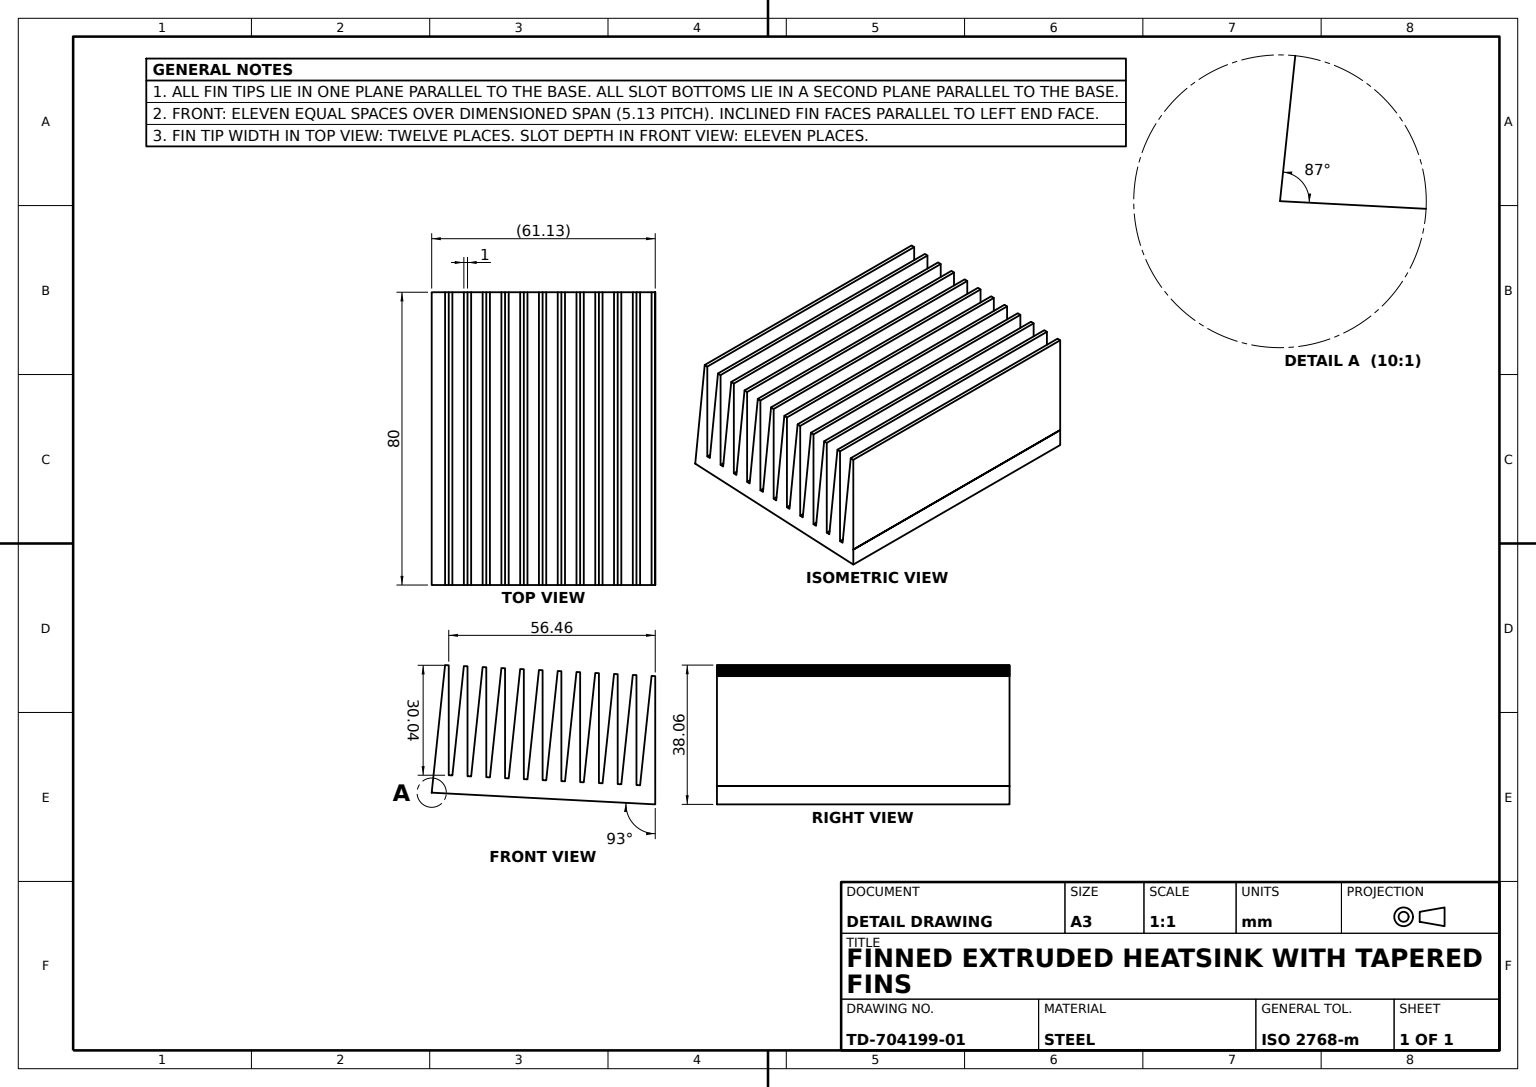
ISO-10303-21;
HEADER;
FILE_DESCRIPTION((''),'2;1');
FILE_NAME('','',(''),(''),'','','');
FILE_SCHEMA(('AUTOMOTIVE_DESIGN'));
ENDSEC;
DATA;
#1=APPLICATION_CONTEXT('');
#2=PRODUCT_CONTEXT('',#1,'mechanical');
#3=PRODUCT('','','',(#2));
#4=PRODUCT_DEFINITION_FORMATION('','',#3);
#5=PRODUCT_DEFINITION_CONTEXT('',#1,'design');
#6=PRODUCT_DEFINITION('','',#4,#5);
#7=PRODUCT_DEFINITION_SHAPE('','',#6);
#8=(LENGTH_UNIT()NAMED_UNIT(*)SI_UNIT(.MILLI.,.METRE.));
#9=(NAMED_UNIT(*)PLANE_ANGLE_UNIT()SI_UNIT($,.RADIAN.));
#10=(NAMED_UNIT(*)SI_UNIT($,.STERADIAN.)SOLID_ANGLE_UNIT());
#11=UNCERTAINTY_MEASURE_WITH_UNIT(LENGTH_MEASURE(1.E-05),#8,'distance_accuracy_value','');
#12=(GEOMETRIC_REPRESENTATION_CONTEXT(3)GLOBAL_UNCERTAINTY_ASSIGNED_CONTEXT((#11))GLOBAL_UNIT_ASSIGNED_CONTEXT((#8,#9,#10))REPRESENTATION_CONTEXT('',''));
#13=CARTESIAN_POINT('',(-19.094272,35.,40.));
#14=VERTEX_POINT('',#13);
#15=CARTESIAN_POINT('',(-19.094272,35.,-40.));
#16=VERTEX_POINT('',#15);
#17=CARTESIAN_POINT('',(-19.094272,35.,0.));
#18=DIRECTION('',(0.,0.,-1.));
#19=VECTOR('',#18,1000.);
#20=LINE('',#17,#19);
#21=EDGE_CURVE('',#14,#16,#20,.T.);
#22=ORIENTED_EDGE('',*,*,#21,.F.);
#23=CARTESIAN_POINT('',(-18.094272,35.,40.));
#24=VERTEX_POINT('',#23);
#25=CARTESIAN_POINT('',(-31.21,35.,40.));
#26=DIRECTION('',(1.,0.,0.));
#27=VECTOR('',#26,1000.);
#28=LINE('',#25,#27);
#29=EDGE_CURVE('',#14,#24,#28,.T.);
#30=ORIENTED_EDGE('',*,*,#29,.T.);
#31=CARTESIAN_POINT('',(-18.094272,35.,-40.));
#32=VERTEX_POINT('',#31);
#33=CARTESIAN_POINT('',(-18.094272,35.,0.));
#34=DIRECTION('',(0.,0.,1.));
#35=VECTOR('',#34,1000.);
#36=LINE('',#33,#35);
#37=EDGE_CURVE('',#32,#24,#36,.T.);
#38=ORIENTED_EDGE('',*,*,#37,.F.);
#39=CARTESIAN_POINT('',(-31.21,35.,-40.));
#40=DIRECTION('',(-1.,0.,0.));
#41=VECTOR('',#40,1000.);
#42=LINE('',#39,#41);
#43=EDGE_CURVE('',#32,#16,#42,.T.);
#44=ORIENTED_EDGE('',*,*,#43,.T.);
#45=EDGE_LOOP('',(#22,#30,#38,#44));
#46=FACE_OUTER_BOUND('',#45,.T.);
#47=CARTESIAN_POINT('',(0.,35.,0.));
#48=DIRECTION('',(0.,-1.,0.));
#49=AXIS2_PLACEMENT_3D('',#47,#48,#18);
#50=PLANE('',#49);
#51=ADVANCED_FACE('',(#46),#50,.F.);
#52=CARTESIAN_POINT('',(27.165728,35.,40.));
#53=VERTEX_POINT('',#52);
#54=CARTESIAN_POINT('',(25.593494,5.,40.));
#55=VERTEX_POINT('',#54);
#56=CARTESIAN_POINT('',(25.262071,-1.323929,40.));
#57=DIRECTION('',(-0.052335956,-0.998629535,0.));
#58=VECTOR('',#57,1000.);
#59=LINE('',#56,#58);
#60=EDGE_CURVE('',#53,#55,#59,.T.);
#61=ORIENTED_EDGE('',*,*,#60,.F.);
#62=CARTESIAN_POINT('',(27.165728,35.,-40.));
#63=VERTEX_POINT('',#62);
#64=CARTESIAN_POINT('',(27.165728,35.,0.));
#65=LINE('',#64,#19);
#66=EDGE_CURVE('',#53,#63,#65,.T.);
#67=ORIENTED_EDGE('',*,*,#66,.T.);
#68=CARTESIAN_POINT('',(25.593494,5.,-40.));
#69=VERTEX_POINT('',#68);
#70=CARTESIAN_POINT('',(27.005834,31.949037,-40.));
#71=LINE('',#70,#58);
#72=EDGE_CURVE('',#63,#69,#71,.T.);
#73=ORIENTED_EDGE('',*,*,#72,.T.);
#74=CARTESIAN_POINT('',(25.593494,5.,-65.));
#75=LINE('',#74,#35);
#76=EDGE_CURVE('',#69,#55,#75,.T.);
#77=ORIENTED_EDGE('',*,*,#76,.T.);
#78=EDGE_LOOP('',(#61,#67,#73,#77));
#79=FACE_OUTER_BOUND('',#78,.T.);
#80=CARTESIAN_POINT('',(25.262071,-1.323929,-65.));
#81=DIRECTION('',(-0.998629535,0.052335956,0.));
#82=AXIS2_PLACEMENT_3D('',#80,#81,#57);
#83=PLANE('',#82);
#84=ADVANCED_FACE('',(#79),#83,.T.);
#85=CARTESIAN_POINT('',(7.605728,35.,-40.));
#86=VERTEX_POINT('',#85);
#87=CARTESIAN_POINT('',(7.605728,35.,40.));
#88=VERTEX_POINT('',#87);
#89=CARTESIAN_POINT('',(7.605728,35.,0.));
#90=LINE('',#89,#35);
#91=EDGE_CURVE('',#86,#88,#90,.T.);
#92=ORIENTED_EDGE('',*,*,#91,.T.);
#93=CARTESIAN_POINT('',(9.177961,5.,40.));
#94=VERTEX_POINT('',#93);
#95=DIRECTION('',(-0.052335956,0.998629535,0.));
#96=VECTOR('',#95,1000.);
#97=LINE('',#93,#96);
#98=EDGE_CURVE('',#94,#88,#97,.T.);
#99=ORIENTED_EDGE('',*,*,#98,.F.);
#100=CARTESIAN_POINT('',(9.177961,5.,-40.));
#101=VERTEX_POINT('',#100);
#102=CARTESIAN_POINT('',(9.177961,5.,-65.));
#103=LINE('',#102,#35);
#104=EDGE_CURVE('',#101,#94,#103,.T.);
#105=ORIENTED_EDGE('',*,*,#104,.F.);
#106=CARTESIAN_POINT('',(7.499409,37.028674,-40.));
#107=LINE('',#106,#96);
#108=EDGE_CURVE('',#101,#86,#107,.T.);
#109=ORIENTED_EDGE('',*,*,#108,.T.);
#110=EDGE_LOOP('',(#92,#99,#105,#109));
#111=FACE_OUTER_BOUND('',#110,.T.);
#112=DIRECTION('',(0.998629535,0.052335956,0.));
#113=AXIS2_PLACEMENT_3D('',#102,#112,#95);
#114=PLANE('',#113);
#115=ADVANCED_FACE('',(#111),#114,.T.);
#116=CARTESIAN_POINT('',(1.465728,35.,-40.));
#117=VERTEX_POINT('',#116);
#118=CARTESIAN_POINT('',(-0.106506,5.,-40.));
#119=VERTEX_POINT('',#118);
#120=CARTESIAN_POINT('',(1.376227,33.292228,-40.));
#121=LINE('',#120,#58);
#122=EDGE_CURVE('',#117,#119,#121,.T.);
#123=ORIENTED_EDGE('',*,*,#122,.T.);
#124=CARTESIAN_POINT('',(-0.106506,5.,40.));
#125=VERTEX_POINT('',#124);
#126=CARTESIAN_POINT('',(-0.106506,5.,-65.));
#127=LINE('',#126,#35);
#128=EDGE_CURVE('',#119,#125,#127,.T.);
#129=ORIENTED_EDGE('',*,*,#128,.T.);
#130=CARTESIAN_POINT('',(1.465728,35.,40.));
#131=VERTEX_POINT('',#130);
#132=CARTESIAN_POINT('',(-0.367535,0.019262,40.));
#133=LINE('',#132,#58);
#134=EDGE_CURVE('',#131,#125,#133,.T.);
#135=ORIENTED_EDGE('',*,*,#134,.F.);
#136=CARTESIAN_POINT('',(1.465728,35.,0.));
#137=LINE('',#136,#19);
#138=EDGE_CURVE('',#131,#117,#137,.T.);
#139=ORIENTED_EDGE('',*,*,#138,.T.);
#140=EDGE_LOOP('',(#123,#129,#135,#139));
#141=FACE_OUTER_BOUND('',#140,.T.);
#142=CARTESIAN_POINT('',(-0.367535,0.019262,-65.));
#143=AXIS2_PLACEMENT_3D('',#142,#81,#57);
#144=PLANE('',#143);
#145=ADVANCED_FACE('',(#141),#144,.T.);
#146=CARTESIAN_POINT('',(24.597961,5.,-40.));
#147=VERTEX_POINT('',#146);
#148=CARTESIAN_POINT('',(-31.21,5.,-40.));
#149=LINE('',#148,#27);
#150=EDGE_CURVE('',#147,#69,#149,.T.);
#151=ORIENTED_EDGE('',*,*,#150,.F.);
#152=CARTESIAN_POINT('',(24.597961,5.,40.));
#153=VERTEX_POINT('',#152);
#154=CARTESIAN_POINT('',(24.597961,5.,-65.));
#155=LINE('',#154,#35);
#156=EDGE_CURVE('',#147,#153,#155,.T.);
#157=ORIENTED_EDGE('',*,*,#156,.T.);
#158=CARTESIAN_POINT('',(0.,5.,40.));
#159=LINE('',#158,#27);
#160=EDGE_CURVE('',#153,#55,#159,.T.);
#161=ORIENTED_EDGE('',*,*,#160,.T.);
#162=ORIENTED_EDGE('',*,*,#76,.F.);
#163=EDGE_LOOP('',(#151,#157,#161,#162));
#164=FACE_OUTER_BOUND('',#163,.T.);
#165=CARTESIAN_POINT('',(0.,5.,-65.));
#166=AXIS2_PLACEMENT_3D('',#165,#48,#18);
#167=PLANE('',#166);
#168=ADVANCED_FACE('',(#164),#167,.F.);
#169=CARTESIAN_POINT('',(-21.662039,5.,40.));
#170=VERTEX_POINT('',#169);
#171=CARTESIAN_POINT('',(-23.234272,35.,40.));
#172=VERTEX_POINT('',#171);
#173=CARTESIAN_POINT('',(-21.341384,-1.118455,40.));
#174=LINE('',#173,#96);
#175=EDGE_CURVE('',#170,#172,#174,.T.);
#176=ORIENTED_EDGE('',*,*,#175,.F.);
#177=CARTESIAN_POINT('',(-21.662039,5.,-40.));
#178=VERTEX_POINT('',#177);
#179=CARTESIAN_POINT('',(-21.662039,5.,-65.));
#180=LINE('',#179,#35);
#181=EDGE_CURVE('',#178,#170,#180,.T.);
#182=ORIENTED_EDGE('',*,*,#181,.F.);
#183=CARTESIAN_POINT('',(-23.234272,35.,-40.));
#184=VERTEX_POINT('',#183);
#185=CARTESIAN_POINT('',(-23.256118,35.416845,-40.));
#186=LINE('',#185,#96);
#187=EDGE_CURVE('',#178,#184,#186,.T.);
#188=ORIENTED_EDGE('',*,*,#187,.T.);
#189=CARTESIAN_POINT('',(-23.234272,35.,0.));
#190=LINE('',#189,#35);
#191=EDGE_CURVE('',#184,#172,#190,.T.);
#192=ORIENTED_EDGE('',*,*,#191,.T.);
#193=EDGE_LOOP('',(#176,#182,#188,#192));
#194=FACE_OUTER_BOUND('',#193,.T.);
#195=CARTESIAN_POINT('',(-21.341384,-1.118455,-65.));
#196=AXIS2_PLACEMENT_3D('',#195,#112,#95);
#197=PLANE('',#196);
#198=ADVANCED_FACE('',(#194),#197,.T.);
#199=ORIENTED_EDGE('',*,*,#128,.F.);
#200=CARTESIAN_POINT('',(-1.102039,5.,-40.));
#201=VERTEX_POINT('',#200);
#202=LINE('',#148,#41);
#203=EDGE_CURVE('',#119,#201,#202,.T.);
#204=ORIENTED_EDGE('',*,*,#203,.T.);
#205=CARTESIAN_POINT('',(-1.102039,5.,40.));
#206=VERTEX_POINT('',#205);
#207=CARTESIAN_POINT('',(-1.102039,5.,-65.));
#208=LINE('',#207,#35);
#209=EDGE_CURVE('',#201,#206,#208,.T.);
#210=ORIENTED_EDGE('',*,*,#209,.T.);
#211=LINE('',#158,#41);
#212=EDGE_CURVE('',#125,#206,#211,.T.);
#213=ORIENTED_EDGE('',*,*,#212,.F.);
#214=EDGE_LOOP('',(#199,#204,#210,#213));
#215=FACE_OUTER_BOUND('',#214,.T.);
#216=DIRECTION('',(0.,1.,0.));
#217=AXIS2_PLACEMENT_3D('',#165,#216,#40);
#218=PLANE('',#217);
#219=ADVANCED_FACE('',(#215),#218,.T.);
#220=CARTESIAN_POINT('',(4.037961,5.,-40.));
#221=VERTEX_POINT('',#220);
#222=CARTESIAN_POINT('',(4.037961,5.,40.));
#223=VERTEX_POINT('',#222);
#224=CARTESIAN_POINT('',(4.037961,5.,-65.));
#225=LINE('',#224,#35);
#226=EDGE_CURVE('',#221,#223,#225,.T.);
#227=ORIENTED_EDGE('',*,*,#226,.F.);
#228=CARTESIAN_POINT('',(2.465728,35.,-40.));
#229=VERTEX_POINT('',#228);
#230=CARTESIAN_POINT('',(2.373488,36.760036,-40.));
#231=LINE('',#230,#96);
#232=EDGE_CURVE('',#221,#229,#231,.T.);
#233=ORIENTED_EDGE('',*,*,#232,.T.);
#234=CARTESIAN_POINT('',(2.465728,35.,40.));
#235=VERTEX_POINT('',#234);
#236=CARTESIAN_POINT('',(2.465728,35.,0.));
#237=LINE('',#236,#35);
#238=EDGE_CURVE('',#229,#235,#237,.T.);
#239=ORIENTED_EDGE('',*,*,#238,.T.);
#240=CARTESIAN_POINT('',(4.288222,0.224736,40.));
#241=LINE('',#240,#96);
#242=EDGE_CURVE('',#223,#235,#241,.T.);
#243=ORIENTED_EDGE('',*,*,#242,.F.);
#244=EDGE_LOOP('',(#227,#233,#239,#243));
#245=FACE_OUTER_BOUND('',#244,.T.);
#246=CARTESIAN_POINT('',(4.288222,0.224736,-65.));
#247=AXIS2_PLACEMENT_3D('',#246,#112,#95);
#248=PLANE('',#247);
#249=ADVANCED_FACE('',(#245),#248,.T.);
#250=CARTESIAN_POINT('',(-11.382039,5.,-40.));
#251=VERTEX_POINT('',#250);
#252=CARTESIAN_POINT('',(-11.382039,5.,40.));
#253=VERTEX_POINT('',#252);
#254=CARTESIAN_POINT('',(-11.382039,5.,-65.));
#255=LINE('',#254,#35);
#256=EDGE_CURVE('',#251,#253,#255,.T.);
#257=ORIENTED_EDGE('',*,*,#256,.F.);
#258=CARTESIAN_POINT('',(-12.954272,35.,-40.));
#259=VERTEX_POINT('',#258);
#260=CARTESIAN_POINT('',(-13.004276,35.954122,-40.));
#261=LINE('',#260,#96);
#262=EDGE_CURVE('',#251,#259,#261,.T.);
#263=ORIENTED_EDGE('',*,*,#262,.T.);
#264=CARTESIAN_POINT('',(-12.954272,35.,40.));
#265=VERTEX_POINT('',#264);
#266=CARTESIAN_POINT('',(-12.954272,35.,0.));
#267=LINE('',#266,#35);
#268=EDGE_CURVE('',#259,#265,#267,.T.);
#269=ORIENTED_EDGE('',*,*,#268,.T.);
#270=CARTESIAN_POINT('',(-11.089542,-0.581178,40.));
#271=LINE('',#270,#96);
#272=EDGE_CURVE('',#253,#265,#271,.T.);
#273=ORIENTED_EDGE('',*,*,#272,.F.);
#274=EDGE_LOOP('',(#257,#263,#269,#273));
#275=FACE_OUTER_BOUND('',#274,.T.);
#276=CARTESIAN_POINT('',(-11.089542,-0.581178,-65.));
#277=AXIS2_PLACEMENT_3D('',#276,#112,#95);
#278=PLANE('',#277);
#279=ADVANCED_FACE('',(#275),#278,.T.);
#280=CARTESIAN_POINT('',(-10.386506,5.,40.));
#281=VERTEX_POINT('',#280);
#282=EDGE_CURVE('',#281,#253,#211,.T.);
#283=ORIENTED_EDGE('',*,*,#282,.F.);
#284=CARTESIAN_POINT('',(-10.386506,5.,-40.));
#285=VERTEX_POINT('',#284);
#286=CARTESIAN_POINT('',(-10.386506,5.,-65.));
#287=LINE('',#286,#35);
#288=EDGE_CURVE('',#285,#281,#287,.T.);
#289=ORIENTED_EDGE('',*,*,#288,.F.);
#290=EDGE_CURVE('',#285,#251,#202,.T.);
#291=ORIENTED_EDGE('',*,*,#290,.T.);
#292=ORIENTED_EDGE('',*,*,#256,.T.);
#293=EDGE_LOOP('',(#283,#289,#291,#292));
#294=FACE_OUTER_BOUND('',#293,.T.);
#295=ADVANCED_FACE('',(#294),#218,.T.);
#296=CARTESIAN_POINT('',(-25.806506,5.,-40.));
#297=VERTEX_POINT('',#296);
#298=CARTESIAN_POINT('',(-26.802039,5.,-40.));
#299=VERTEX_POINT('',#298);
#300=EDGE_CURVE('',#297,#299,#202,.T.);
#301=ORIENTED_EDGE('',*,*,#300,.T.);
#302=CARTESIAN_POINT('',(-26.802039,5.,40.));
#303=VERTEX_POINT('',#302);
#304=CARTESIAN_POINT('',(-26.802039,5.,-65.));
#305=LINE('',#304,#35);
#306=EDGE_CURVE('',#299,#303,#305,.T.);
#307=ORIENTED_EDGE('',*,*,#306,.T.);
#308=CARTESIAN_POINT('',(-25.806506,5.,40.));
#309=VERTEX_POINT('',#308);
#310=LINE('',#308,#41);
#311=EDGE_CURVE('',#309,#303,#310,.T.);
#312=ORIENTED_EDGE('',*,*,#311,.F.);
#313=CARTESIAN_POINT('',(-25.806506,5.,-65.));
#314=LINE('',#313,#35);
#315=EDGE_CURVE('',#297,#309,#314,.T.);
#316=ORIENTED_EDGE('',*,*,#315,.F.);
#317=EDGE_LOOP('',(#301,#307,#312,#316));
#318=FACE_OUTER_BOUND('',#317,.T.);
#319=AXIS2_PLACEMENT_3D('',#313,#216,#40);
#320=PLANE('',#319);
#321=ADVANCED_FACE('',(#318),#320,.T.);
#322=CARTESIAN_POINT('',(5.033494,5.,-40.));
#323=VERTEX_POINT('',#322);
#324=CARTESIAN_POINT('',(5.033494,5.,40.));
#325=VERTEX_POINT('',#324);
#326=CARTESIAN_POINT('',(5.033494,5.,-65.));
#327=LINE('',#326,#35);
#328=EDGE_CURVE('',#323,#325,#327,.T.);
#329=ORIENTED_EDGE('',*,*,#328,.F.);
#330=EDGE_CURVE('',#323,#221,#202,.T.);
#331=ORIENTED_EDGE('',*,*,#330,.T.);
#332=ORIENTED_EDGE('',*,*,#226,.T.);
#333=EDGE_CURVE('',#325,#223,#211,.T.);
#334=ORIENTED_EDGE('',*,*,#333,.F.);
#335=EDGE_LOOP('',(#329,#331,#332,#334));
#336=FACE_OUTER_BOUND('',#335,.T.);
#337=ADVANCED_FACE('',(#336),#218,.T.);
#338=CARTESIAN_POINT('',(-24.234272,35.,-40.));
#339=VERTEX_POINT('',#338);
#340=CARTESIAN_POINT('',(-24.253379,34.635419,-40.));
#341=LINE('',#340,#58);
#342=EDGE_CURVE('',#339,#297,#341,.T.);
#343=ORIENTED_EDGE('',*,*,#342,.T.);
#344=ORIENTED_EDGE('',*,*,#315,.T.);
#345=CARTESIAN_POINT('',(-24.234272,35.,40.));
#346=VERTEX_POINT('',#345);
#347=LINE('',#345,#58);
#348=EDGE_CURVE('',#346,#309,#347,.T.);
#349=ORIENTED_EDGE('',*,*,#348,.F.);
#350=CARTESIAN_POINT('',(-24.234272,35.,0.));
#351=LINE('',#350,#19);
#352=EDGE_CURVE('',#346,#339,#351,.T.);
#353=ORIENTED_EDGE('',*,*,#352,.T.);
#354=EDGE_LOOP('',(#343,#344,#349,#353));
#355=FACE_OUTER_BOUND('',#354,.T.);
#356=CARTESIAN_POINT('',(-24.234272,35.,-65.));
#357=AXIS2_PLACEMENT_3D('',#356,#81,#57);
#358=PLANE('',#357);
#359=ADVANCED_FACE('',(#355),#358,.T.);
#360=CARTESIAN_POINT('',(-28.374272,35.,-40.));
#361=VERTEX_POINT('',#360);
#362=CARTESIAN_POINT('',(-28.382039,35.148207,-40.));
#363=LINE('',#362,#96);
#364=EDGE_CURVE('',#299,#361,#363,.T.);
#365=ORIENTED_EDGE('',*,*,#364,.T.);
#366=CARTESIAN_POINT('',(-28.374272,35.,40.));
#367=VERTEX_POINT('',#366);
#368=CARTESIAN_POINT('',(-28.374272,35.,0.));
#369=LINE('',#368,#35);
#370=EDGE_CURVE('',#361,#367,#369,.T.);
#371=ORIENTED_EDGE('',*,*,#370,.T.);
#372=LINE('',#302,#96);
#373=EDGE_CURVE('',#303,#367,#372,.T.);
#374=ORIENTED_EDGE('',*,*,#373,.F.);
#375=ORIENTED_EDGE('',*,*,#306,.F.);
#376=EDGE_LOOP('',(#365,#371,#374,#375));
#377=FACE_OUTER_BOUND('',#376,.T.);
#378=AXIS2_PLACEMENT_3D('',#304,#112,#95);
#379=PLANE('',#378);
#380=ADVANCED_FACE('',(#377),#379,.T.);
#381=CARTESIAN_POINT('',(-2.674272,35.,-40.));
#382=VERTEX_POINT('',#381);
#383=CARTESIAN_POINT('',(-2.752433,36.491398,-40.));
#384=LINE('',#383,#96);
#385=EDGE_CURVE('',#201,#382,#384,.T.);
#386=ORIENTED_EDGE('',*,*,#385,.T.);
#387=CARTESIAN_POINT('',(-2.674272,35.,40.));
#388=VERTEX_POINT('',#387);
#389=CARTESIAN_POINT('',(-2.674272,35.,0.));
#390=LINE('',#389,#35);
#391=EDGE_CURVE('',#382,#388,#390,.T.);
#392=ORIENTED_EDGE('',*,*,#391,.T.);
#393=CARTESIAN_POINT('',(-0.837699,-0.043902,40.));
#394=LINE('',#393,#96);
#395=EDGE_CURVE('',#206,#388,#394,.T.);
#396=ORIENTED_EDGE('',*,*,#395,.F.);
#397=ORIENTED_EDGE('',*,*,#209,.F.);
#398=EDGE_LOOP('',(#386,#392,#396,#397));
#399=FACE_OUTER_BOUND('',#398,.T.);
#400=CARTESIAN_POINT('',(-0.837699,-0.043902,-65.));
#401=AXIS2_PLACEMENT_3D('',#400,#112,#95);
#402=PLANE('',#401);
#403=ADVANCED_FACE('',(#399),#402,.T.);
#404=CARTESIAN_POINT('',(-6.242039,5.,40.));
#405=VERTEX_POINT('',#404);
#406=CARTESIAN_POINT('',(-7.814272,35.,40.));
#407=VERTEX_POINT('',#406);
#408=CARTESIAN_POINT('',(-5.96362,-0.31254,40.));
#409=LINE('',#408,#96);
#410=EDGE_CURVE('',#405,#407,#409,.T.);
#411=ORIENTED_EDGE('',*,*,#410,.F.);
#412=CARTESIAN_POINT('',(-6.242039,5.,-40.));
#413=VERTEX_POINT('',#412);
#414=CARTESIAN_POINT('',(-6.242039,5.,-65.));
#415=LINE('',#414,#35);
#416=EDGE_CURVE('',#413,#405,#415,.T.);
#417=ORIENTED_EDGE('',*,*,#416,.F.);
#418=CARTESIAN_POINT('',(-7.814272,35.,-40.));
#419=VERTEX_POINT('',#418);
#420=CARTESIAN_POINT('',(-7.878354,36.22276,-40.));
#421=LINE('',#420,#96);
#422=EDGE_CURVE('',#413,#419,#421,.T.);
#423=ORIENTED_EDGE('',*,*,#422,.T.);
#424=CARTESIAN_POINT('',(-7.814272,35.,0.));
#425=LINE('',#424,#35);
#426=EDGE_CURVE('',#419,#407,#425,.T.);
#427=ORIENTED_EDGE('',*,*,#426,.T.);
#428=EDGE_LOOP('',(#411,#417,#423,#427));
#429=FACE_OUTER_BOUND('',#428,.T.);
#430=CARTESIAN_POINT('',(-5.96362,-0.31254,-65.));
#431=AXIS2_PLACEMENT_3D('',#430,#112,#95);
#432=PLANE('',#431);
#433=ADVANCED_FACE('',(#429),#432,.T.);
#434=CARTESIAN_POINT('',(-8.814272,35.,40.));
#435=VERTEX_POINT('',#434);
#436=EDGE_CURVE('',#435,#407,#28,.T.);
#437=ORIENTED_EDGE('',*,*,#436,.T.);
#438=ORIENTED_EDGE('',*,*,#426,.F.);
#439=CARTESIAN_POINT('',(-8.814272,35.,-40.));
#440=VERTEX_POINT('',#439);
#441=EDGE_CURVE('',#419,#440,#42,.T.);
#442=ORIENTED_EDGE('',*,*,#441,.T.);
#443=CARTESIAN_POINT('',(-8.814272,35.,0.));
#444=LINE('',#443,#19);
#445=EDGE_CURVE('',#435,#440,#444,.T.);
#446=ORIENTED_EDGE('',*,*,#445,.F.);
#447=EDGE_LOOP('',(#437,#438,#442,#446));
#448=FACE_OUTER_BOUND('',#447,.T.);
#449=ADVANCED_FACE('',(#448),#50,.F.);
#450=CARTESIAN_POINT('',(-10.619378,0.556538,40.));
#451=LINE('',#450,#58);
#452=EDGE_CURVE('',#435,#281,#451,.T.);
#453=ORIENTED_EDGE('',*,*,#452,.F.);
#454=ORIENTED_EDGE('',*,*,#445,.T.);
#455=CARTESIAN_POINT('',(-8.875615,33.829504,-40.));
#456=LINE('',#455,#58);
#457=EDGE_CURVE('',#440,#285,#456,.T.);
#458=ORIENTED_EDGE('',*,*,#457,.T.);
#459=ORIENTED_EDGE('',*,*,#288,.T.);
#460=EDGE_LOOP('',(#453,#454,#458,#459));
#461=FACE_OUTER_BOUND('',#460,.T.);
#462=CARTESIAN_POINT('',(-10.619378,0.556538,-65.));
#463=AXIS2_PLACEMENT_3D('',#462,#81,#57);
#464=PLANE('',#463);
#465=ADVANCED_FACE('',(#461),#464,.T.);
#466=CARTESIAN_POINT('',(6.605728,35.,40.));
#467=VERTEX_POINT('',#466);
#468=EDGE_CURVE('',#467,#88,#28,.T.);
#469=ORIENTED_EDGE('',*,*,#468,.T.);
#470=ORIENTED_EDGE('',*,*,#91,.F.);
#471=CARTESIAN_POINT('',(6.605728,35.,-40.));
#472=VERTEX_POINT('',#471);
#473=EDGE_CURVE('',#86,#472,#42,.T.);
#474=ORIENTED_EDGE('',*,*,#473,.T.);
#475=CARTESIAN_POINT('',(6.605728,35.,0.));
#476=LINE('',#475,#19);
#477=EDGE_CURVE('',#467,#472,#476,.T.);
#478=ORIENTED_EDGE('',*,*,#477,.F.);
#479=EDGE_LOOP('',(#469,#470,#474,#478));
#480=FACE_OUTER_BOUND('',#479,.T.);
#481=ADVANCED_FACE('',(#480),#50,.F.);
#482=CARTESIAN_POINT('',(4.758386,-0.249376,40.));
#483=LINE('',#482,#58);
#484=EDGE_CURVE('',#467,#325,#483,.T.);
#485=ORIENTED_EDGE('',*,*,#484,.F.);
#486=ORIENTED_EDGE('',*,*,#477,.T.);
#487=CARTESIAN_POINT('',(6.502148,33.02359,-40.));
#488=LINE('',#487,#58);
#489=EDGE_CURVE('',#472,#323,#488,.T.);
#490=ORIENTED_EDGE('',*,*,#489,.T.);
#491=ORIENTED_EDGE('',*,*,#328,.T.);
#492=EDGE_LOOP('',(#485,#486,#490,#491));
#493=FACE_OUTER_BOUND('',#492,.T.);
#494=CARTESIAN_POINT('',(4.758386,-0.249376,-65.));
#495=AXIS2_PLACEMENT_3D('',#494,#81,#57);
#496=PLANE('',#495);
#497=ADVANCED_FACE('',(#493),#496,.T.);
#498=CARTESIAN_POINT('',(19.457961,5.,-40.));
#499=VERTEX_POINT('',#498);
#500=CARTESIAN_POINT('',(19.457961,5.,40.));
#501=VERTEX_POINT('',#500);
#502=CARTESIAN_POINT('',(19.457961,5.,-65.));
#503=LINE('',#502,#35);
#504=EDGE_CURVE('',#499,#501,#503,.T.);
#505=ORIENTED_EDGE('',*,*,#504,.T.);
#506=CARTESIAN_POINT('',(20.453494,5.,40.));
#507=VERTEX_POINT('',#506);
#508=LINE('',#506,#41);
#509=EDGE_CURVE('',#507,#501,#508,.T.);
#510=ORIENTED_EDGE('',*,*,#509,.F.);
#511=CARTESIAN_POINT('',(20.453494,5.,-40.));
#512=VERTEX_POINT('',#511);
#513=CARTESIAN_POINT('',(20.453494,5.,-65.));
#514=LINE('',#513,#35);
#515=EDGE_CURVE('',#512,#507,#514,.T.);
#516=ORIENTED_EDGE('',*,*,#515,.F.);
#517=EDGE_CURVE('',#512,#499,#202,.T.);
#518=ORIENTED_EDGE('',*,*,#517,.T.);
#519=EDGE_LOOP('',(#505,#510,#516,#518));
#520=FACE_OUTER_BOUND('',#519,.T.);
#521=AXIS2_PLACEMENT_3D('',#513,#216,#40);
#522=PLANE('',#521);
#523=ADVANCED_FACE('',(#520),#522,.T.);
#524=CARTESIAN_POINT('',(16.885728,35.,-40.));
#525=VERTEX_POINT('',#524);
#526=CARTESIAN_POINT('',(15.313494,5.,-40.));
#527=VERTEX_POINT('',#526);
#528=CARTESIAN_POINT('',(16.753991,32.486314,-40.));
#529=LINE('',#528,#58);
#530=EDGE_CURVE('',#525,#527,#529,.T.);
#531=ORIENTED_EDGE('',*,*,#530,.T.);
#532=CARTESIAN_POINT('',(15.313494,5.,40.));
#533=VERTEX_POINT('',#532);
#534=CARTESIAN_POINT('',(15.313494,5.,-65.));
#535=LINE('',#534,#35);
#536=EDGE_CURVE('',#527,#533,#535,.T.);
#537=ORIENTED_EDGE('',*,*,#536,.T.);
#538=CARTESIAN_POINT('',(16.885728,35.,40.));
#539=VERTEX_POINT('',#538);
#540=LINE('',#538,#58);
#541=EDGE_CURVE('',#539,#533,#540,.T.);
#542=ORIENTED_EDGE('',*,*,#541,.F.);
#543=CARTESIAN_POINT('',(16.885728,35.,0.));
#544=LINE('',#543,#19);
#545=EDGE_CURVE('',#539,#525,#544,.T.);
#546=ORIENTED_EDGE('',*,*,#545,.T.);
#547=EDGE_LOOP('',(#531,#537,#542,#546));
#548=FACE_OUTER_BOUND('',#547,.T.);
#549=CARTESIAN_POINT('',(16.885728,35.,-65.));
#550=AXIS2_PLACEMENT_3D('',#549,#81,#57);
#551=PLANE('',#550);
#552=ADVANCED_FACE('',(#548),#551,.T.);
#553=CARTESIAN_POINT('',(17.885728,35.,-40.));
#554=VERTEX_POINT('',#553);
#555=CARTESIAN_POINT('',(17.885728,35.,40.));
#556=VERTEX_POINT('',#555);
#557=CARTESIAN_POINT('',(17.885728,35.,0.));
#558=LINE('',#557,#35);
#559=EDGE_CURVE('',#554,#556,#558,.T.);
#560=ORIENTED_EDGE('',*,*,#559,.T.);
#561=LINE('',#500,#96);
#562=EDGE_CURVE('',#501,#556,#561,.T.);
#563=ORIENTED_EDGE('',*,*,#562,.F.);
#564=ORIENTED_EDGE('',*,*,#504,.F.);
#565=CARTESIAN_POINT('',(17.751252,37.56595,-40.));
#566=LINE('',#565,#96);
#567=EDGE_CURVE('',#499,#554,#566,.T.);
#568=ORIENTED_EDGE('',*,*,#567,.T.);
#569=EDGE_LOOP('',(#560,#563,#564,#568));
#570=FACE_OUTER_BOUND('',#569,.T.);
#571=AXIS2_PLACEMENT_3D('',#502,#112,#95);
#572=PLANE('',#571);
#573=ADVANCED_FACE('',(#570),#572,.T.);
#574=CARTESIAN_POINT('',(-30.947753,5.,40.));
#575=VERTEX_POINT('',#574);
#576=CARTESIAN_POINT('',(-30.947753,5.,-40.));
#577=VERTEX_POINT('',#576);
#578=CARTESIAN_POINT('',(-30.947753,5.,-65.));
#579=LINE('',#578,#19);
#580=EDGE_CURVE('',#575,#577,#579,.T.);
#581=ORIENTED_EDGE('',*,*,#580,.T.);
#582=CARTESIAN_POINT('',(-31.21,0.,-40.));
#583=VERTEX_POINT('',#582);
#584=CARTESIAN_POINT('',(-29.379308,34.903981,-40.));
#585=DIRECTION('',(0.05237737,0.998627364,0.));
#586=VECTOR('',#585,1000.);
#587=LINE('',#584,#586);
#588=EDGE_CURVE('',#583,#577,#587,.T.);
#589=ORIENTED_EDGE('',*,*,#588,.F.);
#590=CARTESIAN_POINT('',(-31.21,0.,40.));
#591=VERTEX_POINT('',#590);
#592=LINE('',#590,#35);
#593=EDGE_CURVE('',#583,#591,#592,.T.);
#594=ORIENTED_EDGE('',*,*,#593,.T.);
#595=CARTESIAN_POINT('',(-29.374272,35.,40.));
#596=LINE('',#595,#586);
#597=EDGE_CURVE('',#591,#575,#596,.T.);
#598=ORIENTED_EDGE('',*,*,#597,.T.);
#599=EDGE_LOOP('',(#581,#589,#594,#598));
#600=FACE_OUTER_BOUND('',#599,.T.);
#601=CARTESIAN_POINT('',(-29.374272,35.,-140.145));
#602=DIRECTION('',(0.998627364,-0.05237737,0.));
#603=AXIS2_PLACEMENT_3D('',#601,#602,#585);
#604=PLANE('',#603);
#605=ADVANCED_FACE('',(#600),#604,.F.);
#606=CARTESIAN_POINT('',(-13.954272,35.,-40.));
#607=VERTEX_POINT('',#606);
#608=CARTESIAN_POINT('',(-15.526506,5.,-40.));
#609=VERTEX_POINT('',#608);
#610=CARTESIAN_POINT('',(-14.001537,34.098143,-40.));
#611=LINE('',#610,#58);
#612=EDGE_CURVE('',#607,#609,#611,.T.);
#613=ORIENTED_EDGE('',*,*,#612,.T.);
#614=CARTESIAN_POINT('',(-15.526506,5.,40.));
#615=VERTEX_POINT('',#614);
#616=CARTESIAN_POINT('',(-15.526506,5.,-65.));
#617=LINE('',#616,#35);
#618=EDGE_CURVE('',#609,#615,#617,.T.);
#619=ORIENTED_EDGE('',*,*,#618,.T.);
#620=CARTESIAN_POINT('',(-13.954272,35.,40.));
#621=VERTEX_POINT('',#620);
#622=LINE('',#620,#58);
#623=EDGE_CURVE('',#621,#615,#622,.T.);
#624=ORIENTED_EDGE('',*,*,#623,.F.);
#625=CARTESIAN_POINT('',(-13.954272,35.,0.));
#626=LINE('',#625,#19);
#627=EDGE_CURVE('',#621,#607,#626,.T.);
#628=ORIENTED_EDGE('',*,*,#627,.T.);
#629=EDGE_LOOP('',(#613,#619,#624,#628));
#630=FACE_OUTER_BOUND('',#629,.T.);
#631=CARTESIAN_POINT('',(-13.954272,35.,-65.));
#632=AXIS2_PLACEMENT_3D('',#631,#81,#57);
#633=PLANE('',#632);
#634=ADVANCED_FACE('',(#630),#633,.T.);
#635=ORIENTED_EDGE('',*,*,#515,.T.);
#636=CARTESIAN_POINT('',(22.025728,35.,40.));
#637=VERTEX_POINT('',#636);
#638=LINE('',#636,#58);
#639=EDGE_CURVE('',#637,#507,#638,.T.);
#640=ORIENTED_EDGE('',*,*,#639,.F.);
#641=CARTESIAN_POINT('',(22.025728,35.,-40.));
#642=VERTEX_POINT('',#641);
#643=CARTESIAN_POINT('',(22.025728,35.,0.));
#644=LINE('',#643,#19);
#645=EDGE_CURVE('',#637,#642,#644,.T.);
#646=ORIENTED_EDGE('',*,*,#645,.T.);
#647=CARTESIAN_POINT('',(21.879912,32.217676,-40.));
#648=LINE('',#647,#58);
#649=EDGE_CURVE('',#642,#512,#648,.T.);
#650=ORIENTED_EDGE('',*,*,#649,.T.);
#651=EDGE_LOOP('',(#635,#640,#646,#650));
#652=FACE_OUTER_BOUND('',#651,.T.);
#653=CARTESIAN_POINT('',(22.025728,35.,-65.));
#654=AXIS2_PLACEMENT_3D('',#653,#81,#57);
#655=PLANE('',#654);
#656=ADVANCED_FACE('',(#652),#655,.T.);
#657=ORIENTED_EDGE('',*,*,#391,.F.);
#658=CARTESIAN_POINT('',(-3.674272,35.,-40.));
#659=VERTEX_POINT('',#658);
#660=EDGE_CURVE('',#382,#659,#42,.T.);
#661=ORIENTED_EDGE('',*,*,#660,.T.);
#662=CARTESIAN_POINT('',(-3.674272,35.,40.));
#663=VERTEX_POINT('',#662);
#664=CARTESIAN_POINT('',(-3.674272,35.,0.));
#665=LINE('',#664,#19);
#666=EDGE_CURVE('',#663,#659,#665,.T.);
#667=ORIENTED_EDGE('',*,*,#666,.F.);
#668=EDGE_CURVE('',#663,#388,#28,.T.);
#669=ORIENTED_EDGE('',*,*,#668,.T.);
#670=EDGE_LOOP('',(#657,#661,#667,#669));
#671=FACE_OUTER_BOUND('',#670,.T.);
#672=ADVANCED_FACE('',(#671),#50,.F.);
#673=EDGE_CURVE('',#621,#265,#28,.T.);
#674=ORIENTED_EDGE('',*,*,#673,.T.);
#675=ORIENTED_EDGE('',*,*,#268,.F.);
#676=EDGE_CURVE('',#259,#607,#42,.T.);
#677=ORIENTED_EDGE('',*,*,#676,.T.);
#678=ORIENTED_EDGE('',*,*,#627,.F.);
#679=EDGE_LOOP('',(#674,#675,#677,#678));
#680=FACE_OUTER_BOUND('',#679,.T.);
#681=ADVANCED_FACE('',(#680),#50,.F.);
#682=VERTEX_POINT('',#595);
#683=CARTESIAN_POINT('',(-29.374272,35.,-40.));
#684=VERTEX_POINT('',#683);
#685=CARTESIAN_POINT('',(-29.374272,35.,0.));
#686=LINE('',#685,#19);
#687=EDGE_CURVE('',#682,#684,#686,.T.);
#688=ORIENTED_EDGE('',*,*,#687,.T.);
#689=CARTESIAN_POINT('',(-30.946506,5.,-40.));
#690=VERTEX_POINT('',#689);
#691=CARTESIAN_POINT('',(-29.3793,34.904057,-40.));
#692=LINE('',#691,#58);
#693=EDGE_CURVE('',#684,#690,#692,.T.);
#694=ORIENTED_EDGE('',*,*,#693,.T.);
#695=CARTESIAN_POINT('',(-30.946506,5.,40.));
#696=VERTEX_POINT('',#695);
#697=CARTESIAN_POINT('',(-30.946506,5.,-65.));
#698=LINE('',#697,#35);
#699=EDGE_CURVE('',#690,#696,#698,.T.);
#700=ORIENTED_EDGE('',*,*,#699,.T.);
#701=CARTESIAN_POINT('',(-31.123063,1.631091,40.));
#702=LINE('',#701,#58);
#703=EDGE_CURVE('',#682,#696,#702,.T.);
#704=ORIENTED_EDGE('',*,*,#703,.F.);
#705=EDGE_LOOP('',(#688,#694,#700,#704));
#706=FACE_OUTER_BOUND('',#705,.T.);
#707=CARTESIAN_POINT('',(-31.123063,1.631091,-65.));
#708=AXIS2_PLACEMENT_3D('',#707,#81,#57);
#709=PLANE('',#708);
#710=ADVANCED_FACE('',(#706),#709,.T.);
#711=CARTESIAN_POINT('',(23.025728,35.,-40.));
#712=VERTEX_POINT('',#711);
#713=CARTESIAN_POINT('',(23.025728,35.,40.));
#714=VERTEX_POINT('',#713);
#715=CARTESIAN_POINT('',(23.025728,35.,0.));
#716=LINE('',#715,#35);
#717=EDGE_CURVE('',#712,#714,#716,.T.);
#718=ORIENTED_EDGE('',*,*,#717,.F.);
#719=EDGE_CURVE('',#712,#642,#42,.T.);
#720=ORIENTED_EDGE('',*,*,#719,.T.);
#721=ORIENTED_EDGE('',*,*,#645,.F.);
#722=EDGE_CURVE('',#637,#714,#28,.T.);
#723=ORIENTED_EDGE('',*,*,#722,.T.);
#724=EDGE_LOOP('',(#718,#720,#721,#723));
#725=FACE_OUTER_BOUND('',#724,.T.);
#726=ADVANCED_FACE('',(#725),#50,.F.);
#727=CARTESIAN_POINT('',(30.,0.,-40.));
#728=VERTEX_POINT('',#727);
#729=LINE('',#582,#41);
#730=EDGE_CURVE('',#728,#583,#729,.T.);
#731=ORIENTED_EDGE('',*,*,#730,.F.);
#732=CARTESIAN_POINT('',(30.,0.,40.));
#733=VERTEX_POINT('',#732);
#734=LINE('',#732,#19);
#735=EDGE_CURVE('',#733,#728,#734,.T.);
#736=ORIENTED_EDGE('',*,*,#735,.F.);
#737=LINE('',#590,#27);
#738=EDGE_CURVE('',#591,#733,#737,.T.);
#739=ORIENTED_EDGE('',*,*,#738,.F.);
#740=ORIENTED_EDGE('',*,*,#593,.F.);
#741=EDGE_LOOP('',(#731,#736,#739,#740));
#742=FACE_OUTER_BOUND('',#741,.T.);
#743=CARTESIAN_POINT('',(0.,0.,0.));
#744=AXIS2_PLACEMENT_3D('',#743,#48,#18);
#745=PLANE('',#744);
#746=ADVANCED_FACE('',(#742),#745,.T.);
#747=CARTESIAN_POINT('',(28.165728,35.,40.));
#748=VERTEX_POINT('',#747);
#749=EDGE_CURVE('',#53,#748,#28,.T.);
#750=ORIENTED_EDGE('',*,*,#749,.T.);
#751=CARTESIAN_POINT('',(28.165728,35.,-40.));
#752=VERTEX_POINT('',#751);
#753=CARTESIAN_POINT('',(28.165728,35.,-65.));
#754=LINE('',#753,#35);
#755=EDGE_CURVE('',#752,#748,#754,.T.);
#756=ORIENTED_EDGE('',*,*,#755,.F.);
#757=EDGE_CURVE('',#752,#63,#42,.T.);
#758=ORIENTED_EDGE('',*,*,#757,.T.);
#759=ORIENTED_EDGE('',*,*,#66,.F.);
#760=EDGE_LOOP('',(#750,#756,#758,#759));
#761=FACE_OUTER_BOUND('',#760,.T.);
#762=ADVANCED_FACE('',(#761),#50,.F.);
#763=CARTESIAN_POINT('',(14.317961,5.,-40.));
#764=VERTEX_POINT('',#763);
#765=CARTESIAN_POINT('',(12.745728,35.,-40.));
#766=VERTEX_POINT('',#765);
#767=CARTESIAN_POINT('',(12.625331,37.297312,-40.));
#768=LINE('',#767,#96);
#769=EDGE_CURVE('',#764,#766,#768,.T.);
#770=ORIENTED_EDGE('',*,*,#769,.T.);
#771=CARTESIAN_POINT('',(12.745728,35.,40.));
#772=VERTEX_POINT('',#771);
#773=CARTESIAN_POINT('',(12.745728,35.,0.));
#774=LINE('',#773,#35);
#775=EDGE_CURVE('',#766,#772,#774,.T.);
#776=ORIENTED_EDGE('',*,*,#775,.T.);
#777=CARTESIAN_POINT('',(14.317961,5.,40.));
#778=VERTEX_POINT('',#777);
#779=LINE('',#777,#96);
#780=EDGE_CURVE('',#778,#772,#779,.T.);
#781=ORIENTED_EDGE('',*,*,#780,.F.);
#782=CARTESIAN_POINT('',(14.317961,5.,-65.));
#783=LINE('',#782,#35);
#784=EDGE_CURVE('',#764,#778,#783,.T.);
#785=ORIENTED_EDGE('',*,*,#784,.F.);
#786=EDGE_LOOP('',(#770,#776,#781,#785));
#787=FACE_OUTER_BOUND('',#786,.T.);
#788=AXIS2_PLACEMENT_3D('',#782,#112,#95);
#789=PLANE('',#788);
#790=ADVANCED_FACE('',(#787),#789,.T.);
#791=ORIENTED_EDGE('',*,*,#385,.F.);
#792=ORIENTED_EDGE('',*,*,#203,.F.);
#793=ORIENTED_EDGE('',*,*,#122,.F.);
#794=EDGE_CURVE('',#229,#117,#42,.T.);
#795=ORIENTED_EDGE('',*,*,#794,.F.);
#796=ORIENTED_EDGE('',*,*,#232,.F.);
#797=ORIENTED_EDGE('',*,*,#330,.F.);
#798=ORIENTED_EDGE('',*,*,#489,.F.);
#799=ORIENTED_EDGE('',*,*,#473,.F.);
#800=ORIENTED_EDGE('',*,*,#108,.F.);
#801=CARTESIAN_POINT('',(10.173494,5.,-40.));
#802=VERTEX_POINT('',#801);
#803=EDGE_CURVE('',#802,#101,#202,.T.);
#804=ORIENTED_EDGE('',*,*,#803,.F.);
#805=CARTESIAN_POINT('',(11.745728,35.,-40.));
#806=VERTEX_POINT('',#805);
#807=CARTESIAN_POINT('',(11.62807,32.754952,-40.));
#808=LINE('',#807,#58);
#809=EDGE_CURVE('',#806,#802,#808,.T.);
#810=ORIENTED_EDGE('',*,*,#809,.F.);
#811=EDGE_CURVE('',#766,#806,#42,.T.);
#812=ORIENTED_EDGE('',*,*,#811,.F.);
#813=ORIENTED_EDGE('',*,*,#769,.F.);
#814=EDGE_CURVE('',#527,#764,#202,.T.);
#815=ORIENTED_EDGE('',*,*,#814,.F.);
#816=ORIENTED_EDGE('',*,*,#530,.F.);
#817=EDGE_CURVE('',#554,#525,#42,.T.);
#818=ORIENTED_EDGE('',*,*,#817,.F.);
#819=ORIENTED_EDGE('',*,*,#567,.F.);
#820=ORIENTED_EDGE('',*,*,#517,.F.);
#821=ORIENTED_EDGE('',*,*,#649,.F.);
#822=ORIENTED_EDGE('',*,*,#719,.F.);
#823=CARTESIAN_POINT('',(22.877173,37.834589,-40.));
#824=LINE('',#823,#96);
#825=EDGE_CURVE('',#147,#712,#824,.T.);
#826=ORIENTED_EDGE('',*,*,#825,.F.);
#827=ORIENTED_EDGE('',*,*,#150,.T.);
#828=ORIENTED_EDGE('',*,*,#72,.F.);
#829=ORIENTED_EDGE('',*,*,#757,.F.);
#830=CARTESIAN_POINT('',(28.003095,38.103227,-40.));
#831=LINE('',#830,#96);
#832=EDGE_CURVE('',#728,#752,#831,.T.);
#833=ORIENTED_EDGE('',*,*,#832,.F.);
#834=ORIENTED_EDGE('',*,*,#730,.T.);
#835=ORIENTED_EDGE('',*,*,#588,.T.);
#836=EDGE_CURVE('',#690,#577,#202,.T.);
#837=ORIENTED_EDGE('',*,*,#836,.F.);
#838=ORIENTED_EDGE('',*,*,#693,.F.);
#839=EDGE_CURVE('',#361,#684,#42,.T.);
#840=ORIENTED_EDGE('',*,*,#839,.F.);
#841=ORIENTED_EDGE('',*,*,#364,.F.);
#842=ORIENTED_EDGE('',*,*,#300,.F.);
#843=ORIENTED_EDGE('',*,*,#342,.F.);
#844=EDGE_CURVE('',#184,#339,#42,.T.);
#845=ORIENTED_EDGE('',*,*,#844,.F.);
#846=ORIENTED_EDGE('',*,*,#187,.F.);
#847=CARTESIAN_POINT('',(-20.666506,5.,-40.));
#848=VERTEX_POINT('',#847);
#849=EDGE_CURVE('',#848,#178,#202,.T.);
#850=ORIENTED_EDGE('',*,*,#849,.F.);
#851=CARTESIAN_POINT('',(-19.127458,34.366781,-40.));
#852=LINE('',#851,#58);
#853=EDGE_CURVE('',#16,#848,#852,.T.);
#854=ORIENTED_EDGE('',*,*,#853,.F.);
#855=ORIENTED_EDGE('',*,*,#43,.F.);
#856=CARTESIAN_POINT('',(-16.522039,5.,-40.));
#857=VERTEX_POINT('',#856);
#858=CARTESIAN_POINT('',(-18.130197,35.685483,-40.));
#859=LINE('',#858,#96);
#860=EDGE_CURVE('',#857,#32,#859,.T.);
#861=ORIENTED_EDGE('',*,*,#860,.F.);
#862=EDGE_CURVE('',#609,#857,#202,.T.);
#863=ORIENTED_EDGE('',*,*,#862,.F.);
#864=ORIENTED_EDGE('',*,*,#612,.F.);
#865=ORIENTED_EDGE('',*,*,#676,.F.);
#866=ORIENTED_EDGE('',*,*,#262,.F.);
#867=ORIENTED_EDGE('',*,*,#290,.F.);
#868=ORIENTED_EDGE('',*,*,#457,.F.);
#869=ORIENTED_EDGE('',*,*,#441,.F.);
#870=ORIENTED_EDGE('',*,*,#422,.F.);
#871=CARTESIAN_POINT('',(-5.246506,5.,-40.));
#872=VERTEX_POINT('',#871);
#873=EDGE_CURVE('',#872,#413,#202,.T.);
#874=ORIENTED_EDGE('',*,*,#873,.F.);
#875=CARTESIAN_POINT('',(-3.749694,33.560866,-40.));
#876=LINE('',#875,#58);
#877=EDGE_CURVE('',#659,#872,#876,.T.);
#878=ORIENTED_EDGE('',*,*,#877,.F.);
#879=ORIENTED_EDGE('',*,*,#660,.F.);
#880=EDGE_LOOP('',(#791,#792,#793,#795,#796,#797,#798,#799,#800,#804,#810,#812,#813,#815,#816,#818,#819,#820,#821,#822,#826,#827,#828,#829,#833,#834,#835,#837,#838,#840,#841,#842,#843,#845,#846,#850,#854,#855,#861,#863,#864,#865,#866,#867,#868,#869,#870,#874,#878,#879));
#881=FACE_OUTER_BOUND('',#880,.T.);
#882=AXIS2_PLACEMENT_3D('',#39,#34,#26);
#883=PLANE('',#882);
#884=ADVANCED_FACE('',(#881),#883,.F.);
#885=ORIENTED_EDGE('',*,*,#873,.T.);
#886=ORIENTED_EDGE('',*,*,#416,.T.);
#887=CARTESIAN_POINT('',(-5.246506,5.,40.));
#888=VERTEX_POINT('',#887);
#889=EDGE_CURVE('',#888,#405,#211,.T.);
#890=ORIENTED_EDGE('',*,*,#889,.F.);
#891=CARTESIAN_POINT('',(-5.246506,5.,-65.));
#892=LINE('',#891,#35);
#893=EDGE_CURVE('',#872,#888,#892,.T.);
#894=ORIENTED_EDGE('',*,*,#893,.F.);
#895=EDGE_LOOP('',(#885,#886,#890,#894));
#896=FACE_OUTER_BOUND('',#895,.T.);
#897=ADVANCED_FACE('',(#896),#218,.T.);
#898=ORIENTED_EDGE('',*,*,#784,.T.);
#899=LINE('',#532,#41);
#900=EDGE_CURVE('',#533,#778,#899,.T.);
#901=ORIENTED_EDGE('',*,*,#900,.F.);
#902=ORIENTED_EDGE('',*,*,#536,.F.);
#903=ORIENTED_EDGE('',*,*,#814,.T.);
#904=EDGE_LOOP('',(#898,#901,#902,#903));
#905=FACE_OUTER_BOUND('',#904,.T.);
#906=AXIS2_PLACEMENT_3D('',#534,#216,#40);
#907=PLANE('',#906);
#908=ADVANCED_FACE('',(#905),#907,.T.);
#909=ORIENTED_EDGE('',*,*,#832,.T.);
#910=ORIENTED_EDGE('',*,*,#755,.T.);
#911=CARTESIAN_POINT('',(29.917828,1.567927,40.));
#912=LINE('',#911,#96);
#913=EDGE_CURVE('',#733,#748,#912,.T.);
#914=ORIENTED_EDGE('',*,*,#913,.F.);
#915=ORIENTED_EDGE('',*,*,#735,.T.);
#916=EDGE_LOOP('',(#909,#910,#914,#915));
#917=FACE_OUTER_BOUND('',#916,.T.);
#918=CARTESIAN_POINT('',(29.917828,1.567927,-65.));
#919=AXIS2_PLACEMENT_3D('',#918,#112,#95);
#920=PLANE('',#919);
#921=ADVANCED_FACE('',(#917),#920,.T.);
#922=ORIENTED_EDGE('',*,*,#893,.T.);
#923=CARTESIAN_POINT('',(-5.493456,0.2879,40.));
#924=LINE('',#923,#58);
#925=EDGE_CURVE('',#663,#888,#924,.T.);
#926=ORIENTED_EDGE('',*,*,#925,.F.);
#927=ORIENTED_EDGE('',*,*,#666,.T.);
#928=ORIENTED_EDGE('',*,*,#877,.T.);
#929=EDGE_LOOP('',(#922,#926,#927,#928));
#930=FACE_OUTER_BOUND('',#929,.T.);
#931=CARTESIAN_POINT('',(-5.493456,0.2879,-65.));
#932=AXIS2_PLACEMENT_3D('',#931,#81,#57);
#933=PLANE('',#932);
#934=ADVANCED_FACE('',(#930),#933,.T.);
#935=ORIENTED_EDGE('',*,*,#156,.F.);
#936=ORIENTED_EDGE('',*,*,#825,.T.);
#937=ORIENTED_EDGE('',*,*,#717,.T.);
#938=CARTESIAN_POINT('',(24.791907,1.299289,40.));
#939=LINE('',#938,#96);
#940=EDGE_CURVE('',#153,#714,#939,.T.);
#941=ORIENTED_EDGE('',*,*,#940,.F.);
#942=EDGE_LOOP('',(#935,#936,#937,#941));
#943=FACE_OUTER_BOUND('',#942,.T.);
#944=CARTESIAN_POINT('',(24.791907,1.299289,-65.));
#945=AXIS2_PLACEMENT_3D('',#944,#112,#95);
#946=PLANE('',#945);
#947=ADVANCED_FACE('',(#943),#946,.T.);
#948=ORIENTED_EDGE('',*,*,#580,.F.);
#949=EDGE_CURVE('',#696,#575,#211,.T.);
#950=ORIENTED_EDGE('',*,*,#949,.F.);
#951=ORIENTED_EDGE('',*,*,#699,.F.);
#952=ORIENTED_EDGE('',*,*,#836,.T.);
#953=EDGE_LOOP('',(#948,#950,#951,#952));
#954=FACE_OUTER_BOUND('',#953,.T.);
#955=AXIS2_PLACEMENT_3D('',#165,#216,#34);
#956=PLANE('',#955);
#957=ADVANCED_FACE('',(#954),#956,.T.);
#958=CARTESIAN_POINT('',(11.745728,35.,40.));
#959=VERTEX_POINT('',#958);
#960=CARTESIAN_POINT('',(11.745728,35.,0.));
#961=LINE('',#960,#19);
#962=EDGE_CURVE('',#959,#806,#961,.T.);
#963=ORIENTED_EDGE('',*,*,#962,.T.);
#964=ORIENTED_EDGE('',*,*,#809,.T.);
#965=CARTESIAN_POINT('',(10.173494,5.,40.));
#966=VERTEX_POINT('',#965);
#967=CARTESIAN_POINT('',(10.173494,5.,-65.));
#968=LINE('',#967,#35);
#969=EDGE_CURVE('',#802,#966,#968,.T.);
#970=ORIENTED_EDGE('',*,*,#969,.T.);
#971=LINE('',#958,#58);
#972=EDGE_CURVE('',#959,#966,#971,.T.);
#973=ORIENTED_EDGE('',*,*,#972,.F.);
#974=EDGE_LOOP('',(#963,#964,#970,#973));
#975=FACE_OUTER_BOUND('',#974,.T.);
#976=CARTESIAN_POINT('',(11.745728,35.,-65.));
#977=AXIS2_PLACEMENT_3D('',#976,#81,#57);
#978=PLANE('',#977);
#979=ADVANCED_FACE('',(#975),#978,.T.);
#980=ORIENTED_EDGE('',*,*,#794,.T.);
#981=ORIENTED_EDGE('',*,*,#138,.F.);
#982=EDGE_CURVE('',#131,#235,#28,.T.);
#983=ORIENTED_EDGE('',*,*,#982,.T.);
#984=ORIENTED_EDGE('',*,*,#238,.F.);
#985=EDGE_LOOP('',(#980,#981,#983,#984));
#986=FACE_OUTER_BOUND('',#985,.T.);
#987=ADVANCED_FACE('',(#986),#50,.F.);
#988=ORIENTED_EDGE('',*,*,#844,.T.);
#989=ORIENTED_EDGE('',*,*,#352,.F.);
#990=EDGE_CURVE('',#346,#172,#28,.T.);
#991=ORIENTED_EDGE('',*,*,#990,.T.);
#992=ORIENTED_EDGE('',*,*,#191,.F.);
#993=EDGE_LOOP('',(#988,#989,#991,#992));
#994=FACE_OUTER_BOUND('',#993,.T.);
#995=ADVANCED_FACE('',(#994),#50,.F.);
#996=ORIENTED_EDGE('',*,*,#860,.T.);
#997=ORIENTED_EDGE('',*,*,#37,.T.);
#998=CARTESIAN_POINT('',(-16.522039,5.,40.));
#999=VERTEX_POINT('',#998);
#1000=LINE('',#998,#96);
#1001=EDGE_CURVE('',#999,#24,#1000,.T.);
#1002=ORIENTED_EDGE('',*,*,#1001,.F.);
#1003=CARTESIAN_POINT('',(-16.522039,5.,-65.));
#1004=LINE('',#1003,#35);
#1005=EDGE_CURVE('',#857,#999,#1004,.T.);
#1006=ORIENTED_EDGE('',*,*,#1005,.F.);
#1007=EDGE_LOOP('',(#996,#997,#1002,#1006));
#1008=FACE_OUTER_BOUND('',#1007,.T.);
#1009=AXIS2_PLACEMENT_3D('',#1003,#112,#95);
#1010=PLANE('',#1009);
#1011=ADVANCED_FACE('',(#1008),#1010,.T.);
#1012=ORIENTED_EDGE('',*,*,#962,.F.);
#1013=EDGE_CURVE('',#959,#772,#28,.T.);
#1014=ORIENTED_EDGE('',*,*,#1013,.T.);
#1015=ORIENTED_EDGE('',*,*,#775,.F.);
#1016=ORIENTED_EDGE('',*,*,#811,.T.);
#1017=EDGE_LOOP('',(#1012,#1014,#1015,#1016));
#1018=FACE_OUTER_BOUND('',#1017,.T.);
#1019=ADVANCED_FACE('',(#1018),#50,.F.);
#1020=ORIENTED_EDGE('',*,*,#618,.F.);
#1021=ORIENTED_EDGE('',*,*,#862,.T.);
#1022=ORIENTED_EDGE('',*,*,#1005,.T.);
#1023=LINE('',#614,#41);
#1024=EDGE_CURVE('',#615,#999,#1023,.T.);
#1025=ORIENTED_EDGE('',*,*,#1024,.F.);
#1026=EDGE_LOOP('',(#1020,#1021,#1022,#1025));
#1027=FACE_OUTER_BOUND('',#1026,.T.);
#1028=AXIS2_PLACEMENT_3D('',#616,#216,#40);
#1029=PLANE('',#1028);
#1030=ADVANCED_FACE('',(#1027),#1029,.T.);
#1031=CARTESIAN_POINT('',(-20.666506,5.,40.));
#1032=VERTEX_POINT('',#1031);
#1033=CARTESIAN_POINT('',(-20.87122,1.093814,40.));
#1034=LINE('',#1033,#58);
#1035=EDGE_CURVE('',#14,#1032,#1034,.T.);
#1036=ORIENTED_EDGE('',*,*,#1035,.F.);
#1037=ORIENTED_EDGE('',*,*,#21,.T.);
#1038=ORIENTED_EDGE('',*,*,#853,.T.);
#1039=CARTESIAN_POINT('',(-20.666506,5.,-65.));
#1040=LINE('',#1039,#35);
#1041=EDGE_CURVE('',#848,#1032,#1040,.T.);
#1042=ORIENTED_EDGE('',*,*,#1041,.T.);
#1043=EDGE_LOOP('',(#1036,#1037,#1038,#1042));
#1044=FACE_OUTER_BOUND('',#1043,.T.);
#1045=CARTESIAN_POINT('',(-20.87122,1.093814,-65.));
#1046=AXIS2_PLACEMENT_3D('',#1045,#81,#57);
#1047=PLANE('',#1046);
#1048=ADVANCED_FACE('',(#1044),#1047,.T.);
#1049=ORIENTED_EDGE('',*,*,#181,.T.);
#1050=EDGE_CURVE('',#1032,#170,#211,.T.);
#1051=ORIENTED_EDGE('',*,*,#1050,.F.);
#1052=ORIENTED_EDGE('',*,*,#1041,.F.);
#1053=ORIENTED_EDGE('',*,*,#849,.T.);
#1054=EDGE_LOOP('',(#1049,#1051,#1052,#1053));
#1055=FACE_OUTER_BOUND('',#1054,.T.);
#1056=ADVANCED_FACE('',(#1055),#218,.T.);
#1057=ORIENTED_EDGE('',*,*,#212,.T.);
#1058=ORIENTED_EDGE('',*,*,#395,.T.);
#1059=ORIENTED_EDGE('',*,*,#668,.F.);
#1060=ORIENTED_EDGE('',*,*,#925,.T.);
#1061=ORIENTED_EDGE('',*,*,#889,.T.);
#1062=ORIENTED_EDGE('',*,*,#410,.T.);
#1063=ORIENTED_EDGE('',*,*,#436,.F.);
#1064=ORIENTED_EDGE('',*,*,#452,.T.);
#1065=ORIENTED_EDGE('',*,*,#282,.T.);
#1066=ORIENTED_EDGE('',*,*,#272,.T.);
#1067=ORIENTED_EDGE('',*,*,#673,.F.);
#1068=ORIENTED_EDGE('',*,*,#623,.T.);
#1069=ORIENTED_EDGE('',*,*,#1024,.T.);
#1070=ORIENTED_EDGE('',*,*,#1001,.T.);
#1071=ORIENTED_EDGE('',*,*,#29,.F.);
#1072=ORIENTED_EDGE('',*,*,#1035,.T.);
#1073=ORIENTED_EDGE('',*,*,#1050,.T.);
#1074=ORIENTED_EDGE('',*,*,#175,.T.);
#1075=ORIENTED_EDGE('',*,*,#990,.F.);
#1076=ORIENTED_EDGE('',*,*,#348,.T.);
#1077=ORIENTED_EDGE('',*,*,#311,.T.);
#1078=ORIENTED_EDGE('',*,*,#373,.T.);
#1079=EDGE_CURVE('',#682,#367,#28,.T.);
#1080=ORIENTED_EDGE('',*,*,#1079,.F.);
#1081=ORIENTED_EDGE('',*,*,#703,.T.);
#1082=ORIENTED_EDGE('',*,*,#949,.T.);
#1083=ORIENTED_EDGE('',*,*,#597,.F.);
#1084=ORIENTED_EDGE('',*,*,#738,.T.);
#1085=ORIENTED_EDGE('',*,*,#913,.T.);
#1086=ORIENTED_EDGE('',*,*,#749,.F.);
#1087=ORIENTED_EDGE('',*,*,#60,.T.);
#1088=ORIENTED_EDGE('',*,*,#160,.F.);
#1089=ORIENTED_EDGE('',*,*,#940,.T.);
#1090=ORIENTED_EDGE('',*,*,#722,.F.);
#1091=ORIENTED_EDGE('',*,*,#639,.T.);
#1092=ORIENTED_EDGE('',*,*,#509,.T.);
#1093=ORIENTED_EDGE('',*,*,#562,.T.);
#1094=EDGE_CURVE('',#539,#556,#28,.T.);
#1095=ORIENTED_EDGE('',*,*,#1094,.F.);
#1096=ORIENTED_EDGE('',*,*,#541,.T.);
#1097=ORIENTED_EDGE('',*,*,#900,.T.);
#1098=ORIENTED_EDGE('',*,*,#780,.T.);
#1099=ORIENTED_EDGE('',*,*,#1013,.F.);
#1100=ORIENTED_EDGE('',*,*,#972,.T.);
#1101=LINE('',#965,#41);
#1102=EDGE_CURVE('',#966,#94,#1101,.T.);
#1103=ORIENTED_EDGE('',*,*,#1102,.T.);
#1104=ORIENTED_EDGE('',*,*,#98,.T.);
#1105=ORIENTED_EDGE('',*,*,#468,.F.);
#1106=ORIENTED_EDGE('',*,*,#484,.T.);
#1107=ORIENTED_EDGE('',*,*,#333,.T.);
#1108=ORIENTED_EDGE('',*,*,#242,.T.);
#1109=ORIENTED_EDGE('',*,*,#982,.F.);
#1110=ORIENTED_EDGE('',*,*,#134,.T.);
#1111=EDGE_LOOP('',(#1057,#1058,#1059,#1060,#1061,#1062,#1063,#1064,#1065,#1066,#1067,#1068,#1069,#1070,#1071,#1072,#1073,#1074,#1075,#1076,#1077,#1078,#1080,#1081,#1082,#1083,#1084,#1085,#1086,#1087,#1088,#1089,#1090,#1091,#1092,#1093,#1095,#1096,#1097,#1098,#1099,#1100,#1103,#1104,#1105,#1106,#1107,#1108,#1109,#1110));
#1112=FACE_OUTER_BOUND('',#1111,.T.);
#1113=AXIS2_PLACEMENT_3D('',#25,#18,#40);
#1114=PLANE('',#1113);
#1115=ADVANCED_FACE('',(#1112),#1114,.F.);
#1116=ORIENTED_EDGE('',*,*,#687,.F.);
#1117=ORIENTED_EDGE('',*,*,#1079,.T.);
#1118=ORIENTED_EDGE('',*,*,#370,.F.);
#1119=ORIENTED_EDGE('',*,*,#839,.T.);
#1120=EDGE_LOOP('',(#1116,#1117,#1118,#1119));
#1121=FACE_OUTER_BOUND('',#1120,.T.);
#1122=ADVANCED_FACE('',(#1121),#50,.F.);
#1123=ORIENTED_EDGE('',*,*,#104,.T.);
#1124=ORIENTED_EDGE('',*,*,#1102,.F.);
#1125=ORIENTED_EDGE('',*,*,#969,.F.);
#1126=ORIENTED_EDGE('',*,*,#803,.T.);
#1127=EDGE_LOOP('',(#1123,#1124,#1125,#1126));
#1128=FACE_OUTER_BOUND('',#1127,.T.);
#1129=AXIS2_PLACEMENT_3D('',#967,#216,#40);
#1130=PLANE('',#1129);
#1131=ADVANCED_FACE('',(#1128),#1130,.T.);
#1132=ORIENTED_EDGE('',*,*,#545,.F.);
#1133=ORIENTED_EDGE('',*,*,#1094,.T.);
#1134=ORIENTED_EDGE('',*,*,#559,.F.);
#1135=ORIENTED_EDGE('',*,*,#817,.T.);
#1136=EDGE_LOOP('',(#1132,#1133,#1134,#1135));
#1137=FACE_OUTER_BOUND('',#1136,.T.);
#1138=ADVANCED_FACE('',(#1137),#50,.F.);
#1139=CLOSED_SHELL('',(#51,#84,#115,#145,#168,#198,#219,#249,#279,#295,#321,#337,#359,#380,#403,#433,#449,#465,#481,#497,#523,#552,#573,#605,#634,#656,#672,#681,#710,#726,#746,#762,#790,#884,#897,#908,#921,#934,#947,#957,#979,#987,#995,#1011,#1019,#1030,#1048,#1056,#1115,#1122,#1131,#1138));
#1140=MANIFOLD_SOLID_BREP('',#1139);
#1141=ADVANCED_BREP_SHAPE_REPRESENTATION('',(#1140),#12);
#1142=SHAPE_DEFINITION_REPRESENTATION(#7,#1141);
ENDSEC;
END-ISO-10303-21;
